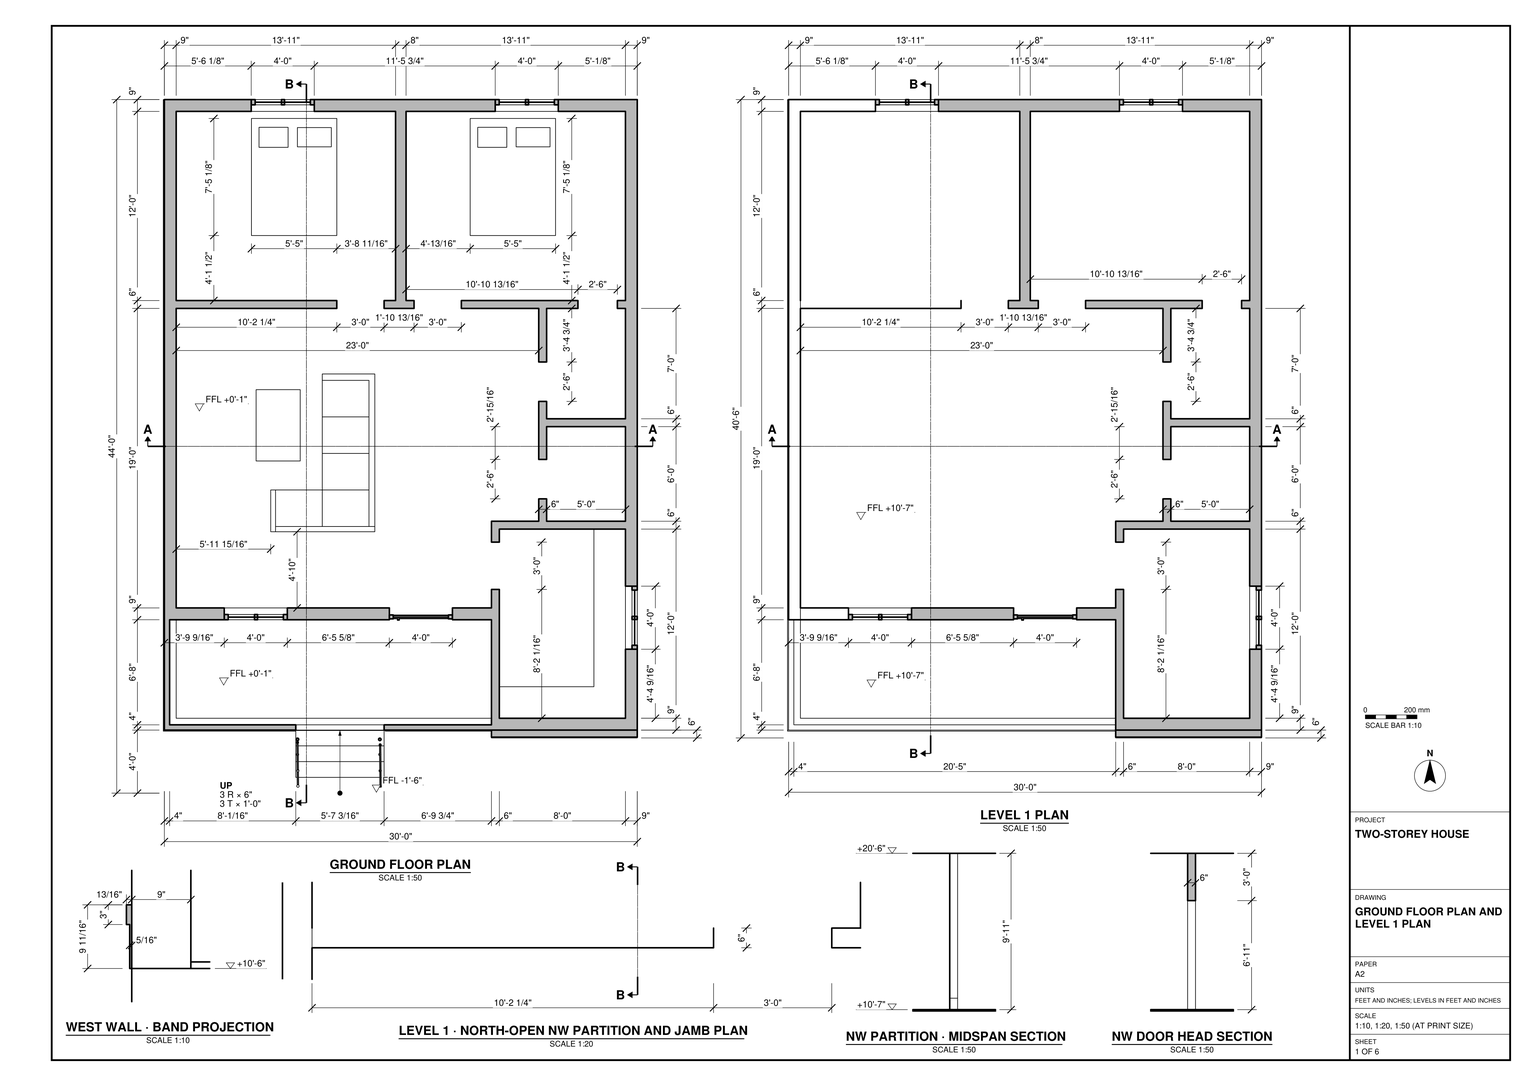
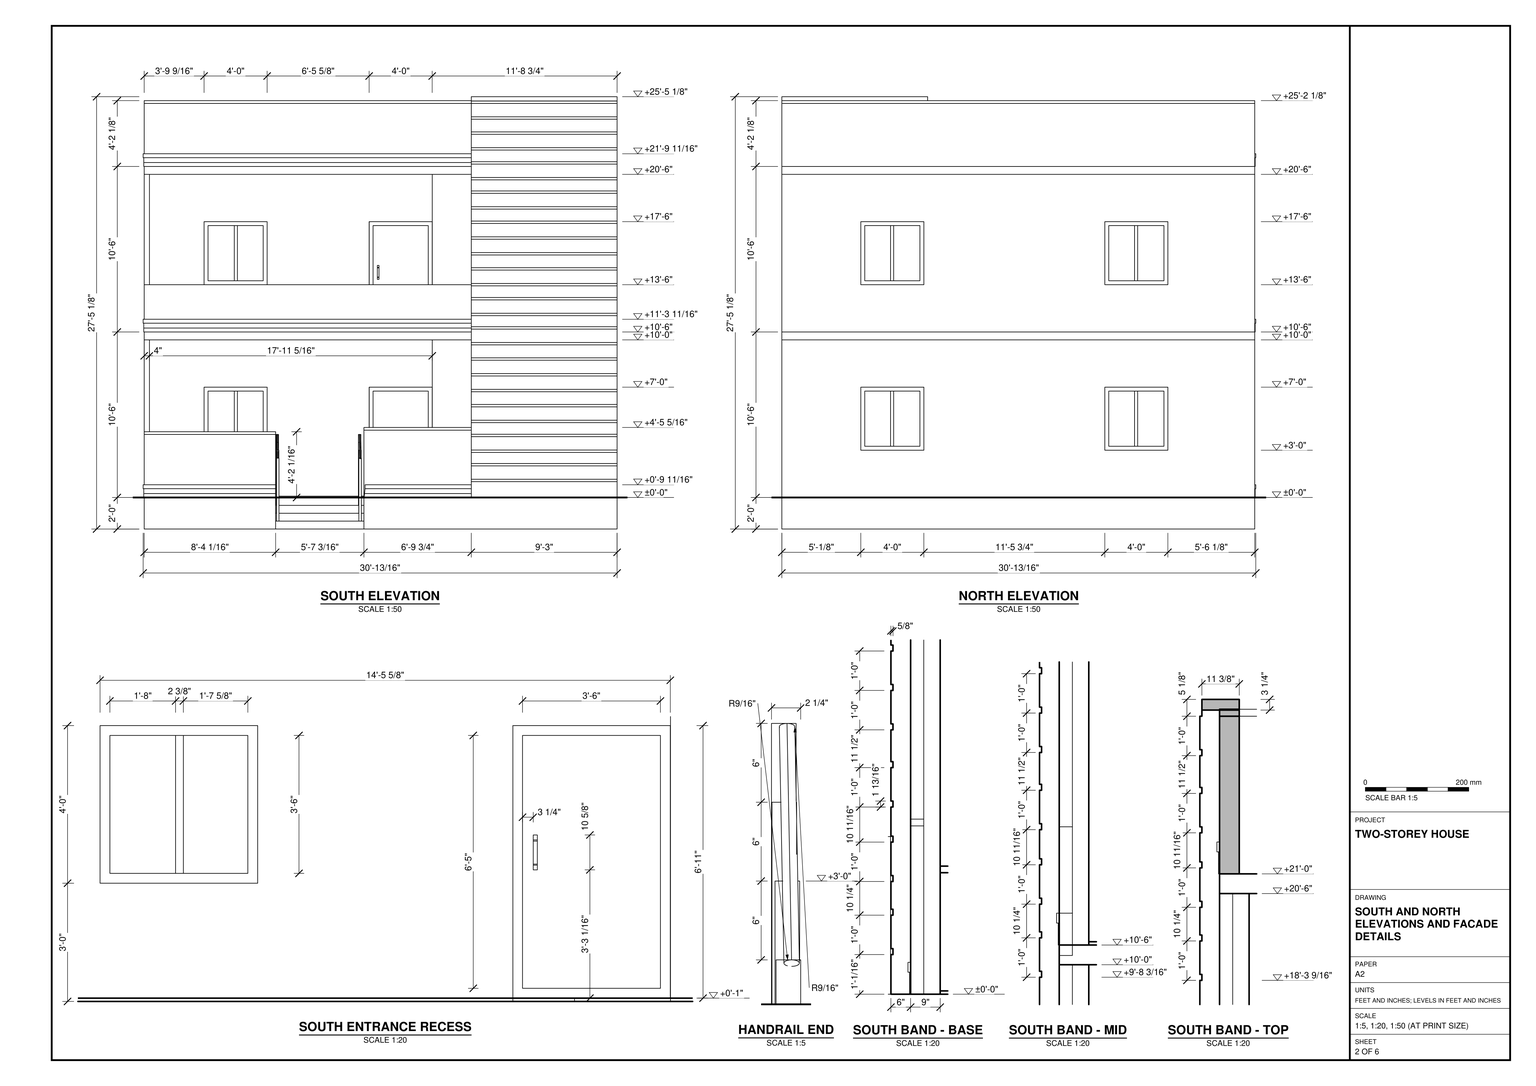
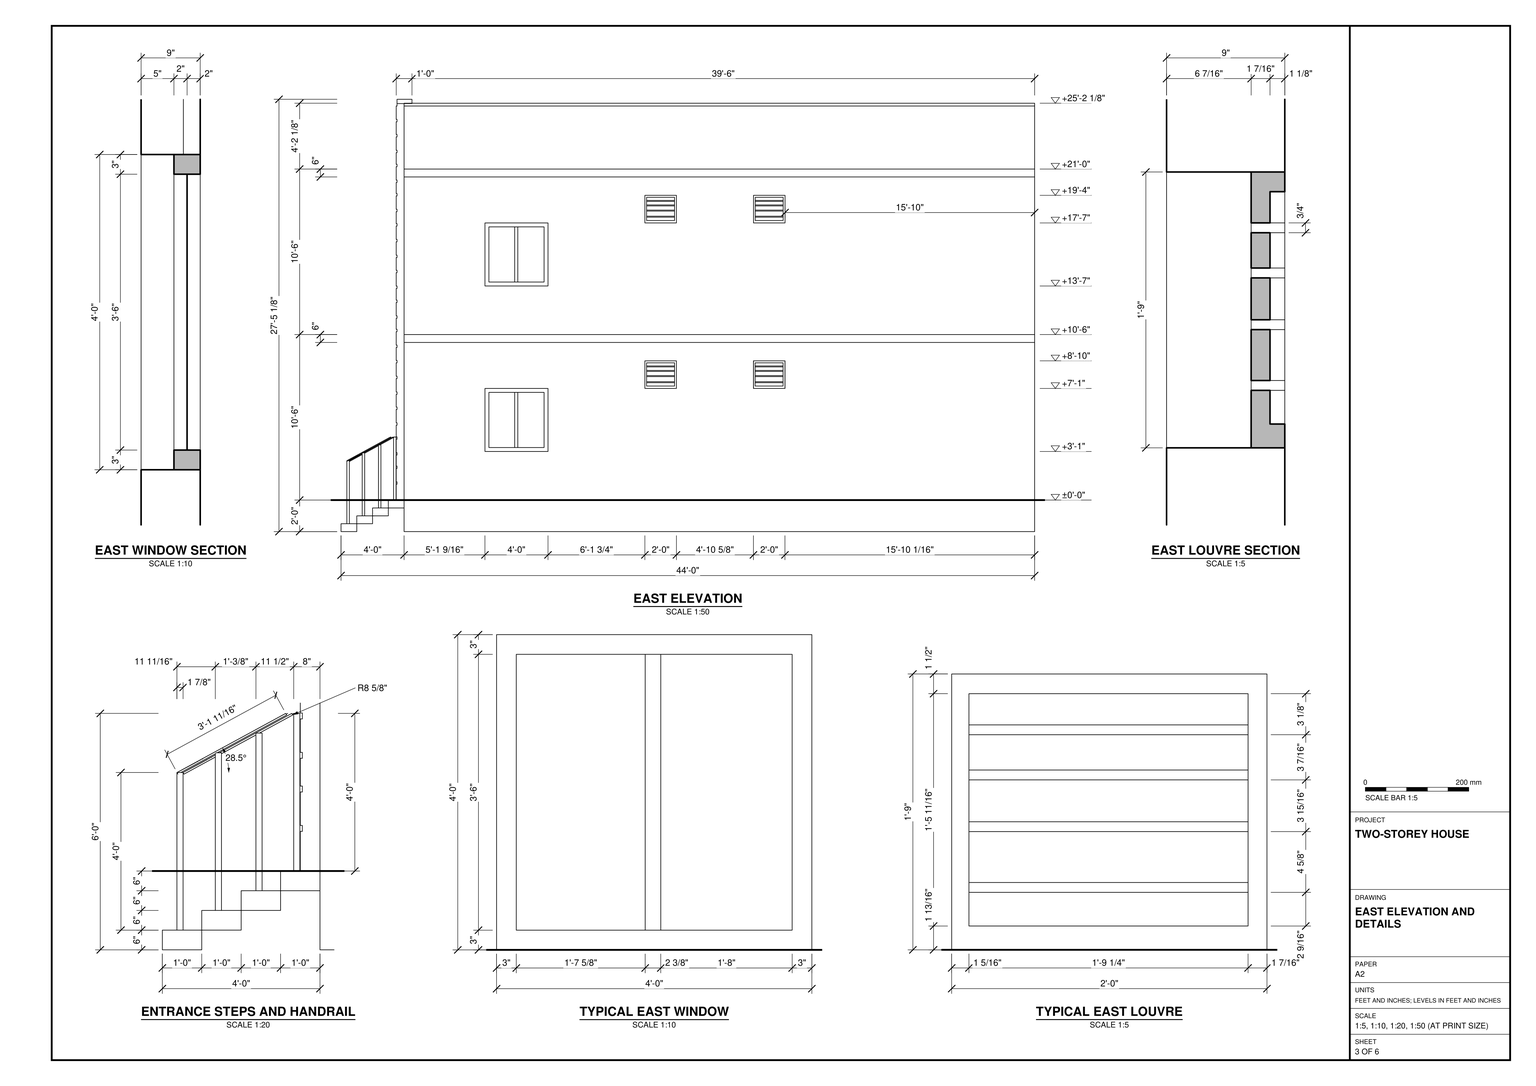
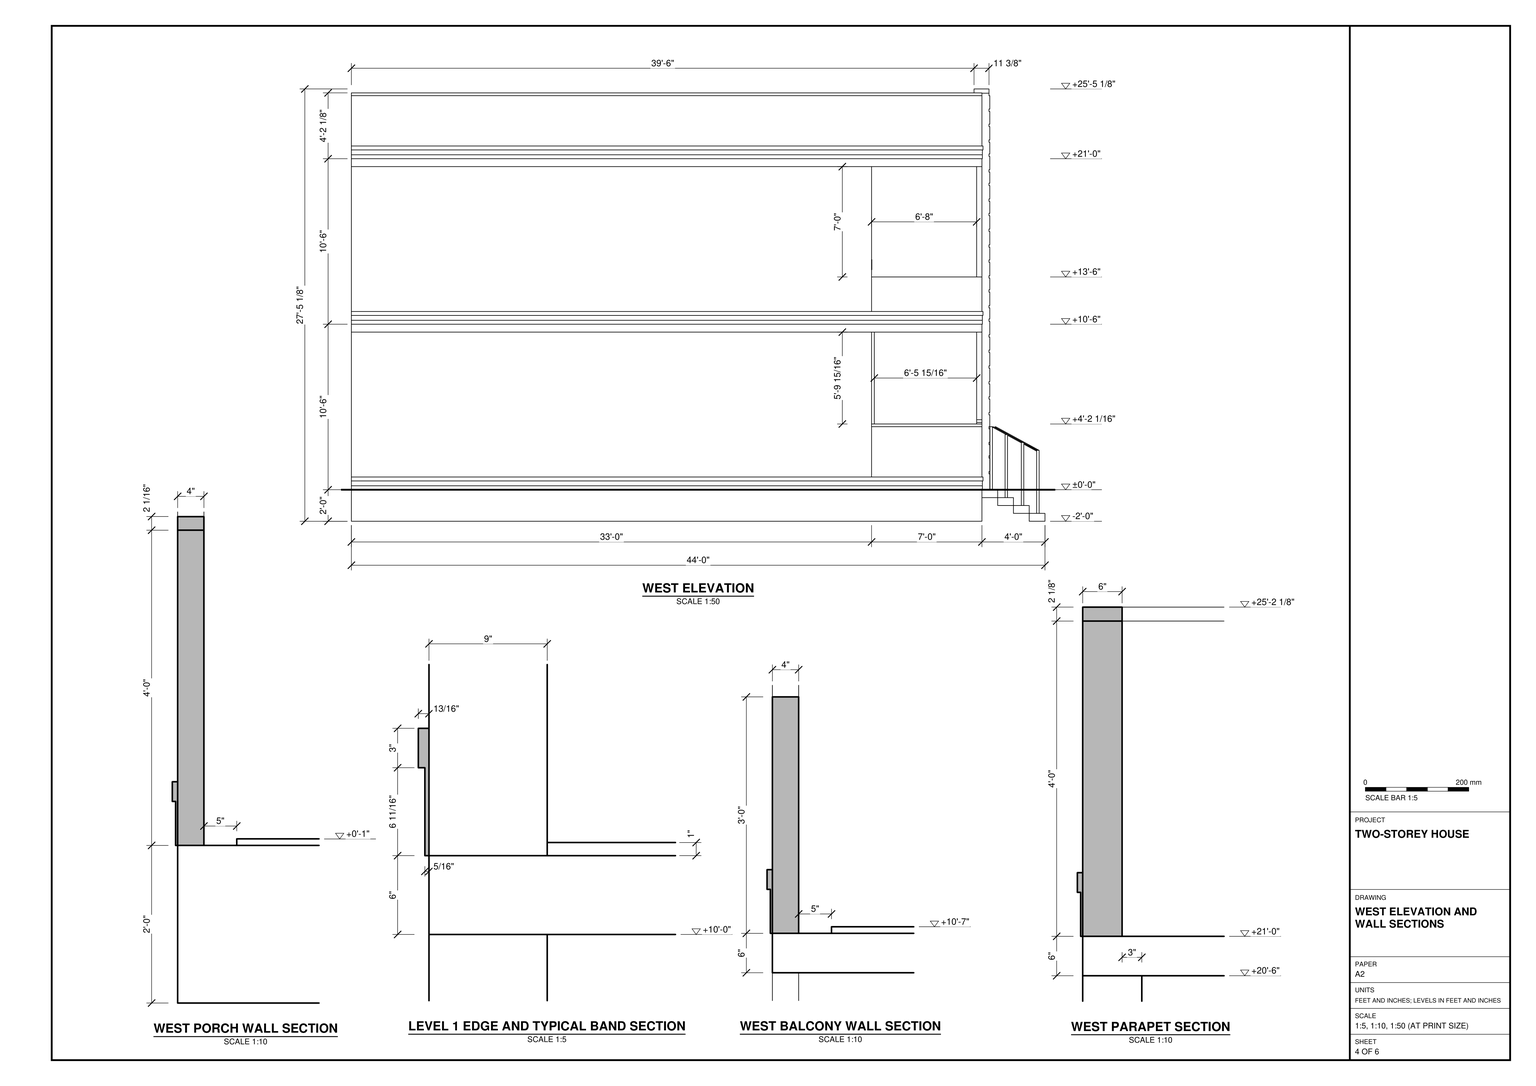
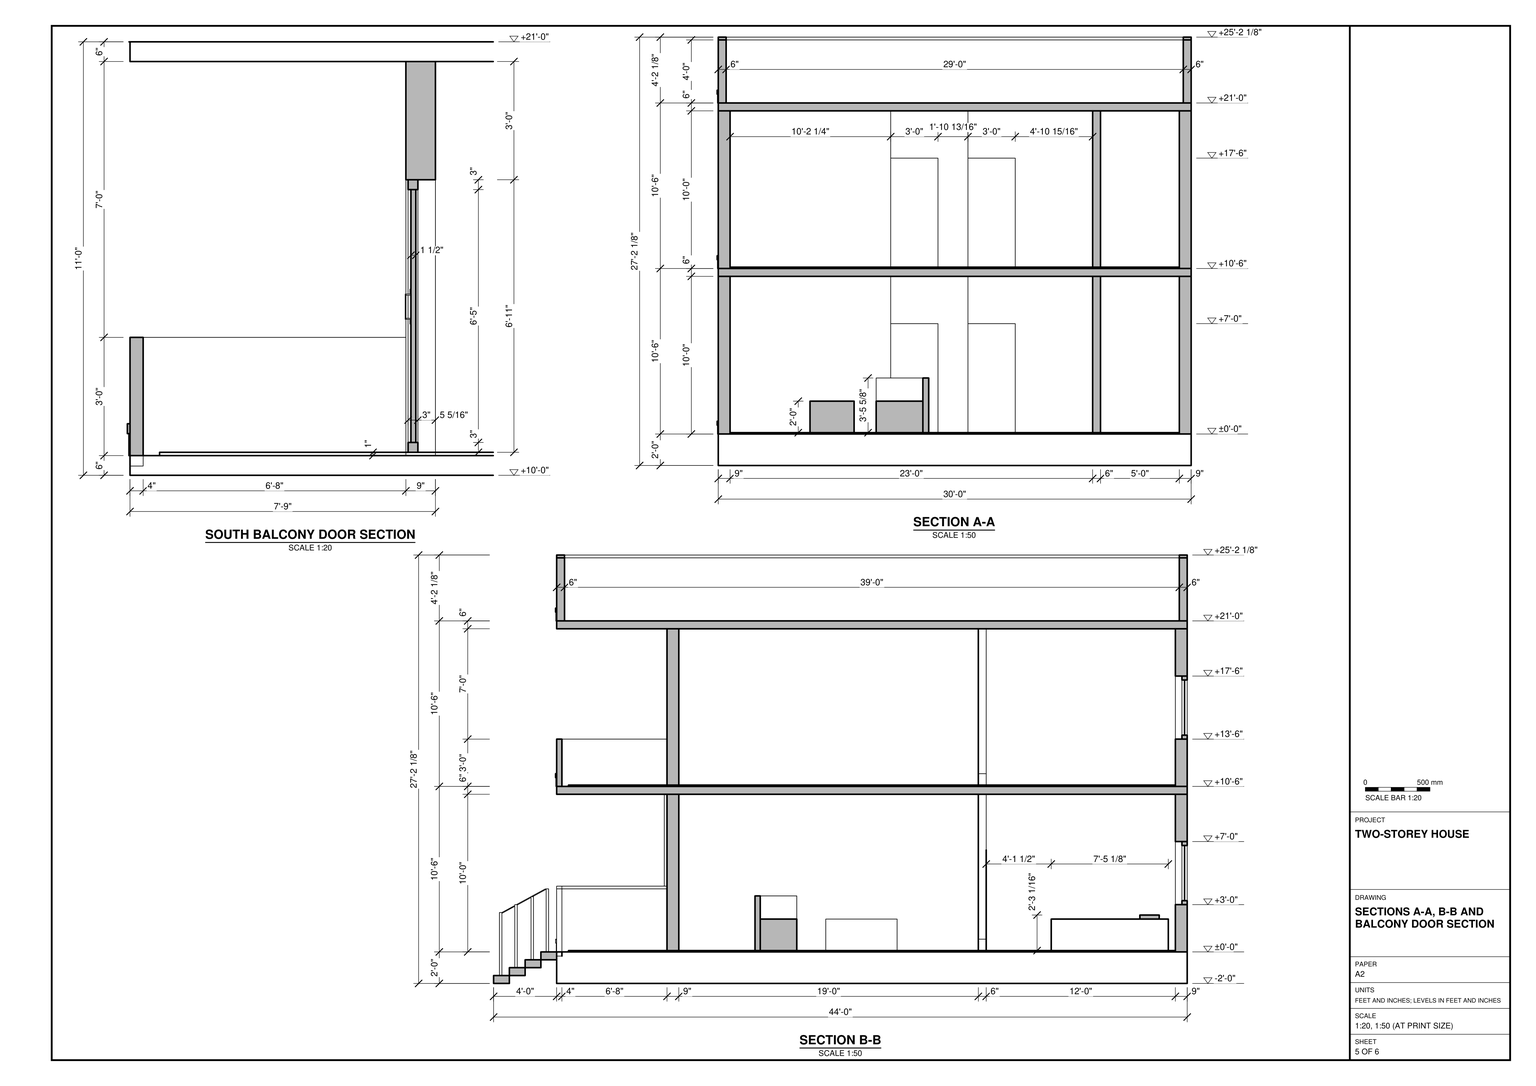
Build the house in SketchUp using task_files/diagram_01.pdf. Work in feet and inches. The overall model measures 30'-13/16" east to west, 44'-0" north to south including the entrance steps, and 27'-5 1/8" from its lowest point to its highest point. Set the ground floor at ±0'-0" and the upper floor at +10'-6".

Use the two plans separately to lay out the walls and openings. Follow the drawn wall thicknesses, including the 9" exterior walls, the 8" dividing wall between the rear rooms and the 6" partitions where indicated. Follow the upper-floor partition and jamb detail at the northwest room. Model the floor slabs, flat roof and parapets. On the south side, form the recessed porch and the balcony above it, with the entrance steps and handrails leading through the gap in the porch wall. Carry the horizontal bands across the full-height bay beside the recess as shown in elevation.

Fit the doors, window units and east-wall louvres to their openings. Place the beds in the rear ground-floor rooms and arrange the L-shaped sofa and low table to match their plan footprints. Decor and loose items may be any suitable library components. Keep walls, slabs, roof, and each furniture or joinery piece in separate groups or components, and use components for repeated parts. Save one SketchUp model as output_files/two_storey_house_with_a_recessed_porch_and_balcony.skp.

# SketchUp Ruby script. Lengths in inches.
U = 1.inch
M = Sketchup.active_model
def pt(a) = Geom::Point3d.new(a.map { |v| v * U })
def face(e, loops, mat)
  f = e.add_face(loops[0].map { |a| pt(a) })
  loops[1..].each { |l| e.add_face(l.map { |a| pt(a) }).erase! }
  f.material = f.back_material = mat if mat
  f
end
# faces: each face lists its corners as indices into pts; further lists are holes
def faces(e, pts, list, mat = nil) = list.each { |f| face(e, (f[0].is_a?(Array) ? f : [f]).map { |l| l.map { |i| pts[i] } }, mat) }
# xy, xz, yz: faces in a plane at the given z, y or x. An outline is a flat list of corners, or four numbers for a rectangle; further outlines are holes
def ring(l) = l.size == 4 ? [[l[0], l[1]], [l[2], l[1]], [l[2], l[3]], [l[0], l[3]]] : l.each_slice(2).to_a
def flat(e, list, mat, &to3) = list.each { |f| face(e, (f[0].is_a?(Array) ? f : [f]).map { |l| ring(l).map { |u, v| to3.(u, v) } }, mat) }
def xy(e, z, list, mat = nil) = flat(e, list, mat) { |x, y| [x, y, z] }
def xz(e, y, list, mat = nil) = flat(e, list, mat) { |x, z| [x, y, z] }
def yz(e, x, list, mat = nil) = flat(e, list, mat) { |y, z| [x, y, z] }
def lines(e, pts, list) = list.each { |a, b| e.add_line(pt(pts[a]), pt(pts[b])) }
# prism: a flat outline (further loops are holes) pulled along v
def prism(e, loops, v, mat = nil)
  f = face(e, loops, mat); d = Geom::Vector3d.new(v.map { |x| x * U })
  f.pushpull(f.normal.samedirection?(d) ? d.length : -d.length)
end
def box(e, o, s, mat = nil) = prism(e, [[o, [o[0] + s[0], o[1], o[2]], [o[0] + s[0], o[1] + s[1], o[2]], [o[0], o[1] + s[1], o[2]]]], [0, 0, s[2]], mat)
def at(x, y, z, deg = 0) = Geom::Transformation.translation(pt([x, y, z])) * Geom::Transformation.rotation(ORIGIN, Z_AXIS, deg.degrees)
def axes(o, x, y, z) = Geom::Transformation.new([*x, 0, *y, 0, *z, 0, *pt(o).to_a, 1])
def part(name) = M.definitions.add(name)
# library, detail: a bought-in or finely detailed component or shape, given as its bounding box
def library(name, o, s) = part(name).tap { |d| box(d.entities, o, s) }
def detail(e, o, s) = box(e.add_group.entities, o, s)
def put(e, d, t, mat = nil) = e.add_instance(d, t).tap { |i| i.material = mat if mat }
def group(e, t, mat = nil) = e.add_group.tap { |g| g.transformation = t; g.material = mat if mat }.entities
root = M.entities
M.materials.add("A01_Blush_Petal").color = [255, 204, 204]
M.materials.add("A02_Rose_Quartz").color = [255, 153, 153]
M.materials.add("C07_Caramel_Shine").color = [153, 76, 0]
M.materials.add("C08_Toffee_Ember").color = [102, 51, 0]
M.materials.add("D01_Frost_White").color = [255, 242, 206]
M.materials.add("D02_Buttercup_Glow").color = [255, 229, 155]
M.materials.add("D03_Lemon_Mist").color = [255, 216, 101]
M.materials.add("Forest_Floor_01_1K").color = [106, 91, 72]
M.materials.add("Glass_Basic_01").color = [161, 173, 186]
M.materials["Glass_Basic_01"].alpha = 0.25
M.materials.add("Glass_Safety_01").color = [204, 235, 244]
M.materials["Glass_Safety_01"].alpha = 0.25
M.materials.add("H02_Aqua_Frost").color = [153, 255, 255]
M.materials.add("H07_Deep_Teal").color = [0, 153, 153]
M.materials.add("M01_Silver_Fog").color = [224, 224, 224]
M.materials.add("M05_Graphite_Haze").color = [114, 114, 114]
M.materials.add("M09_Shadow_Night").color = [0, 0, 0]
M.materials.add("Marble_06_1K").color = [165, 150, 147]
M.materials.add("Metal_06_1K").color = [238, 236, 231]
M.materials.add("Plywood_01_1K").color = [125, 96, 64]
c1 = part("Group\#5")
box(c1.entities,[-7.22,0,-6],[67.22,12,6])
c2 = part("Group\#9")
g1 = group(c2.entities,at(3,2,3),"Glass_Safety_01")
xz(g1,0,[[0,0,42,42]])
g2 = group(c2.entities,at(0,4,0),"Plywood_01_1K")
xy(g2,0,[[0,-4,48,0]])
xy(g2,3,[[3,-4,23,0],[23,-4,25.375,0],[25.375,-4,45,0]])
xy(g2,45,[[3,-4,23,0],[23,-4,25.375,0],[25.375,-4,45,0]])
xy(g2,48,[[0,-4,48,0]])
xz(g2,-4,[[[0,0,48,48],[3,3,45,45]],[23,3,25.375,45]],"Plywood_01_1K")
xz(g2,0,[[[0,0,48,48],[3,3,45,45]],[23,3,25.375,45]])
yz(g2,0,[[-4,0,0,48]])
yz(g2,3,[[-4,3,0,45]])
yz(g2,23,[[-4,3,0,45]])
yz(g2,25.375,[[-4,3,0,45]])
yz(g2,45,[[-4,3,0,45]])
yz(g2,48,[[-4,0,0,48]])
c3 = part("Group\#10")
xy(c3.entities,0,[[-0.25,0,2.3125,24]])
xy(c3.entities,1.8125,[[1.1875,1.3125,2.3125,22.5625]])
xy(c3.entities,4.375,[[-0.25,1.3125,1.1875,22.5625]])
xy(c3.entities,5.125,[[-0.25,1.3125,1.1875,22.5625]])
xy(c3.entities,9,[[-0.25,1.3125,1.1875,22.5625]])
xy(c3.entities,9.75,[[-0.25,1.3125,1.1875,22.5625]])
xy(c3.entities,12.9375,[[-0.25,1.3125,1.1875,22.5625]])
xy(c3.entities,13.6875,[[-0.25,1.3125,1.1875,22.5625]])
xy(c3.entities,16.375,[[-0.25,1.3125,1.1875,22.5625]])
xy(c3.entities,17.125,[[-0.25,1.3125,1.1875,22.5625]])
xy(c3.entities,19.5,[[1.1875,1.3125,2.3125,22.5625]])
xy(c3.entities,21,[[-0.25,0,2.3125,24]])
xz(c3.entities,0,[[-0.25,0,2.3125,21]])
xz(c3.entities,1.3125,[[1.1875,1.8125,2.3125,4.375],[-0.25,4.375,2.3125,5.125],[1.1875,5.125,2.3125,9],[-0.25,9,2.3125,9.75],[1.1875,9.75,2.3125,12.9375],
  [-0.25,12.9375,2.3125,13.6875],[1.1875,13.6875,2.3125,16.375],[-0.25,16.375,2.3125,17.125],[1.1875,17.125,2.3125,19.5]])
xz(c3.entities,22.5625,[[1.1875,1.8125,2.3125,4.375],[-0.25,4.375,2.3125,5.125],[1.1875,5.125,2.3125,9],[-0.25,9,2.3125,9.75],[1.1875,9.75,2.3125,12.9375],
  [-0.25,12.9375,2.3125,13.6875],[1.1875,13.6875,2.3125,16.375],[-0.25,16.375,2.3125,17.125],[1.1875,17.125,2.3125,19.5]])
xz(c3.entities,24,[[-0.25,0,2.3125,21]])
yz(c3.entities,-0.25,[[[0,0,24,21],[1.3125,16.375,22.5625,17.125],[1.3125,12.9375,22.5625,13.6875],[1.3125,9,22.5625,9.75],[1.3125,4.375,22.5625,5.125]]])
yz(c3.entities,1.1875,[[1.3125,1.8125,22.5625,4.375],[1.3125,5.125,22.5625,9],[1.3125,9.75,22.5625,12.9375],[1.3125,13.6875,22.5625,16.375],[1.3125,17.125,22.5625,19.5]])
yz(c3.entities,2.3125,[[[0,0,24,21],[1.3125,1.8125,22.5625,19.5]]])
c4 = part("Group\#16")
g3 = group(c4.entities,at(0,3.875,0),"Plywood_01_1K")
prism(g3,[[[0,0,83],[48,0,83],[48,0,0],[0,0,0]],[[45,0,3],[45,0,80],[3,0,80],[3,0,3]]],[0,-3,0])
g4 = group(c4.entities,at(6.26,1.75,47.9375),"Metal_06_1K")
xy(g4,-8.875,[[0,-0.3125,1.25,0]])
xy(g4,-7.4375,[[0,-1.75,1.25,-1.5],[0,-1.5,1.25,-0.3125],[0,-0.3125,1.25,0]])
xy(g4,-7.125,[[0,-1.75,1.25,-1.5],[0,-1.5,1.25,0]])
xy(g4,-0.125,[[0,-1.75,1.25,-1.5],[0,-1.5,1.25,0]])
xy(g4,0.25,[[0,-1.75,1.25,-1.5],[0,-1.5,1.25,-0.3125],[0,-0.3125,1.25,0]])
xy(g4,1.75,[[0,-0.3125,1.25,0]])
xz(g4,-1.75,[[0,-7.4375,1.25,-7.125],[0,-7.125,1.25,-0.125],[0,-0.125,1.25,0.25]])
xz(g4,-1.5,[[0,-7.4375,1.25,-7.125],[0,-7.125,1.25,-0.125],[0,-0.125,1.25,0.25]])
xz(g4,-0.3125,[[0,-8.875,1.25,-7.4375],[0,0.25,1.25,1.75]])
xz(g4,0,[[0,-7.4375,1.25,-7.125],[0,-0.125,1.25,0.25],[0,0.25,1.25,1.75]])
yz(g4,0,[[-0.3125,-8.875,0,-7.4375],[-1.75,-7.4375,-1.5,-7.125],[-1.5,-7.4375,0,-7.125],[-1.75,-7.125,-1.5,-0.125],[-1.75,-0.125,-1.5,0.25],
  [-1.5,-0.125,0,0.25],[-0.3125,0.25,0,1.75]])
yz(g4,1.25,[[-0.3125,-8.875,0,-7.4375],[-1.75,-7.4375,-1.5,-7.125],[-1.5,-7.4375,0,-7.125],[-1.75,-7.125,-1.5,-0.125],[-1.75,-0.125,-1.5,0.25],
  [-1.5,-0.125,0,0.25],[-0.3125,0.25,0,1.75]])
g5 = group(c4.entities,at(3,3.25,3))
box(g5,[0,-1.5,0],[42,1.5,77],"Plywood_01_1K")
c5 = part("Group\#19")
prism(c5.entities,[[[0.9375,1.875,0],[1.18,1.84,0],[1.41,1.75,0],[1.6,1.6,0],[1.75,1.41,0],[1.84,1.18,0],[1.875,0.9375,0],[1.84,0.69,0],[1.75,0.47,0],[1.6,0.27,0],[1.41,0.125,0],[1.18,0.03,0],[0.9375,0,0],[0.69,0.03,0],[0.47,0.125,0],[0.27,0.27,0],[0.125,0.47,0],[0.03,0.69,0],[0,0.9375,0],[0.03,1.18,0],[0.125,1.41,0],[0.27,1.6,0],[0.47,1.75,0],[0.69,1.84,0]]],[0,0,48])
c6 = part("Group\#20")
prism(c6.entities,[[[1.24,-32.84,-18.46],[1.36,-32.86,-18.42],[1.46,-32.89,-18.37],[1.51,-32.92,-18.31],[1.53,-32.95,-18.24],[1.51,-32.99,-18.18],[1.45,-33.02,-18.12],[1.36,-33.05,-18.07],[1.23,-33.07,-18.03],[1.09,-33.09,-18.01],[0.9375,-33.09,-18],[0.79,-33.09,-18.01],[0.64,-33.08,-18.03],[0.52,-33.06,-18.07],[0.43,-33.03,-18.125],[0.37,-33,-18.1875],[0.35,-32.96,-18.25],[0.375,-32.93,-18.3125],[0.44,-32.9,-18.375],[0.53,-32.87,-18.42],[0.65,-32.84,-18.46],[0.8,-32.83,-18.49],[0.95,-32.82,-18.49],[1.1,-32.83,-18.49]]],[-0.35,33.09,18])
c7 = part("Group\#22")
xy(c7.entities,0,[[-0.3125,-0.3125,0,480],[0,-0.3125,249,0]],"C08_Toffee_Ember")
xy(c7.entities,6.69,[[-0.8125,-0.8125,-0.3125,480],[-0.3125,-0.8125,249,-0.3125]],"C08_Toffee_Ember")
xy(c7.entities,9.69,[[-0.8125,-0.8125,249,0],[-0.8125,0,0,480]],"C08_Toffee_Ember")
xz(c7.entities,-0.8125,[[-0.8125,6.69,249,9.69]],"C08_Toffee_Ember")
xz(c7.entities,-0.3125,[[-0.3125,0,249,3]],"C08_Toffee_Ember")
xz(c7.entities,-0.3125,[[-0.3125,3,249,6.69]],"D03_Lemon_Mist")
xz(c7.entities,480,[[-0.3125,3,0,6.69]])
xz(c7.entities,480,[[-0.3125,0,0,3],[-0.8125,6.69,0,9.69]],"C08_Toffee_Ember")
yz(c7.entities,-0.8125,[[-0.8125,6.69,480,9.69]],"C08_Toffee_Ember")
yz(c7.entities,-0.3125,[[-0.3125,0,480,3]],"C08_Toffee_Ember")
yz(c7.entities,-0.3125,[[-0.3125,3,480,6.69]],"D03_Lemon_Mist")
yz(c7.entities,249,[[-0.3125,3,0,6.69]])
yz(c7.entities,249,[[-0.3125,0,0,3],[-0.8125,6.69,0,9.69]],"C08_Toffee_Ember")
c8 = part("Group\#28")
box(c8.entities,[0,0,0],[35.5625,27.8125,24])
c9 = part("Group\#30")
box(c9.entities,[0,0,0],[65,89.125,24])
g6 = group(c9.entities,at(5.77,67.15,24),"A02_Rose_Quartz")
box(g6,[29.21,0.36,0],[25.82,14.69,3.0625])
box(g6,[0,0,0],[22.125,15.25,3.0625])
xy(root,1,[[70.66,252.86,104.22,307.17]])
xy(root,25,[[70.66,252.86,104.22,307.17]],"A01_Blush_Petal")
xy(root,252,[[6.8125,54,354.8125,522]])
xz(root,252.86,[[70.66,1,104.22,25]],"Glass_Basic_01")
xz(root,307.17,[[70.66,1,104.22,25]],"Glass_Basic_01")
xz(root,375,[[9.8125,0,132.08,77.62]])
yz(root,70.66,[[252.86,1,307.17,25]],"Glass_Basic_01")
yz(root,104.22,[[252.86,1,307.17,25]],"Glass_Basic_01")
p = [[100.87,48,0],[108.08,48,0]]
lines(root,p,[[0,1]])
g7 = group(root,at(0.8125,48,0))
xy(g7,0,[[0,0,100.05,0,100.05,4,4,4,4,84,0,84],[249,0,360,0,360,480,0,480,0,84,45.59,84,45.59,93,9,93,9,321,131.27,321,131.27,327,9,327,9,471,176,471,176,327,167.27,327,167.27,321,190.08,321,190.08,327,184,327,184,471,351,471,351,327,344.84,327,344.84,321,351,321,351,237,291,237,291,321,314.84,321,314.84,327,226.08,327,226.08,321,285,321,285,206.03,291,206.03,291,231,351,231,351,159,291,159,291,176.03,285,176.03,285,159,249,159,249,143.07,255,143.07,255,153,351,153,351,9,255,9,255,107.07,249,107.07,249,93,219.3,93,219.3,84,249,84],[167.27,0,249,4],[255,9,351,153],[45.59,84,93.59,93],
  [93.59,84,171.3,93],[171.3,84,219.3,93],[9,93,249,93,249,159,285,159,285,321,9,321],[249,107.07,255,143.07],[291,159,351,231],
  [285,176.03,291,206.03],[291,237,351,321],[131.27,321,167.27,327],[190.08,321,226.08,327],[314.84,321,344.84,327],
  [9,327,176,471],[184,327,351,471]])
xy(g7,0,[[100.05,0,167.27,4],[4,4,249,84]],"D02_Buttercup_Glow")
g8 = group(root,at(0.8125,48,120),"D01_Frost_White")
box(g8,[0,0,0],[360,480,6])
g9 = group(root,at(0.8125,48,0),"D01_Frost_White")
xy(g9,0,[[0,0,0,84,4,84,4,4,100.05,4,100.05,0],[45.59,84,171.3,93],[285,250.22,291,280.22]])
xy(g9,36,[[45.59,84,93.59,93],[66.125,471,114.125,480],[251.875,471,299.875,480]])
xy(g9,37,[[351,61.5625,360,109.5625]])
xy(g9,48,[[0,0,0,84,4,84,4,4,100.05,4,100.05,0]],"M05_Graphite_Haze")
xy(g9,50.0625,[[0,0,100.05,0,100.05,4,4,4,4,81.9375,0,81.9375],[0,81.9375,4,84]],"M05_Graphite_Haze")
xy(g9,51.25,[[167.27,0,249,4]],"M05_Graphite_Haze")
xy(g9,53.3125,[[167.27,0,249,4]],"M05_Graphite_Haze")
xy(g9,84,[[45.59,84,93.59,93],[171.3,84,219.3,93],[249,107.07,255,143.07],[285,176.03,291,206.03],[285,250.22,291,280.22],
  [131.27,321,167.27,327],[190.08,321,226.08,327],[314.84,321,344.84,327],[66.125,471,114.125,480],[251.875,471,299.875,480]])
xy(g9,85,[[351,61.5625,360,109.5625],[351,183.3125,360,207.3125],[351,266,360,290]])
xy(g9,106,[[351,183.3125,360,207.3125],[351,266,360,290]])
xy(g9,120,[[[249,0,360,0,360,480,0,480,0,84,219.3,84,219.3,93,9,93,9,321,131.27,321,131.27,327,9,327,9,471,176,471,176,327,131.27,327,131.27,321,285,321,285,206.03,291,206.03,291,231,351,231,351,159,291,159,291,206.03,285,206.03,285,159,249,159,249,143.07,255,143.07,255,153,351,153,351,9,255,9,255,143.07,249,143.07,249,93,219.3,93,219.3,84,249,84],[291,237,291,321,314.84,321,314.84,327,184,327,184,471,351,471,351,327,314.84,327,314.84,321,351,321,351,237]]])
xy(g9,120,[[0,81.9375,4,84]],"M05_Graphite_Haze")
xz(g9,0,[[0,0,100.05,48],[167.27,0,249,51.25],[249,0,360,120]])
xz(g9,0,[[0,48,100.05,50.0625],[167.27,51.25,249,53.3125]],"M05_Graphite_Haze")
xz(g9,4,[[100.05,-3.1875,167.27,0],[4,0,100.05,48],[167.27,0,249,51.25]])
xz(g9,4,[[4,48,100.05,50.0625],[167.27,51.25,249,53.3125]],"M05_Graphite_Haze")
xz(g9,9,[[255,0,351,120]])
xz(g9,61.5625,[[351,37,360,85]])
xz(g9,81.9375,[[0,50.0625,4,120]],"M05_Graphite_Haze")
xz(g9,84,[[[4,0,171.3,0,171.3,84,219.3,84,219.3,120,4,120],[45.59,36,93.59,84]],[219.3,0,249,120]])
xz(g9,84,[[0,48,4,50.0625],[0,50.0625,4,120]],"M05_Graphite_Haze")
xz(g9,93,[[[9,0,9,120,219.3,120,219.3,84,171.3,84,171.3,0],[45.59,36,93.59,84]],[219.3,0,249,120]])
xz(g9,107.07,[[249,0,255,84]])
xz(g9,109.5625,[[351,37,360,85]])
xz(g9,143.07,[[249,0,255,84]])
xz(g9,153,[[255,0,351,120]])
xz(g9,159,[[249,0,285,120],[291,0,351,120]])
xz(g9,176.03,[[285,0,291,84]])
xz(g9,183.3125,[[351,85,360,106]])
xz(g9,206.03,[[285,0,291,84]])
xz(g9,207.3125,[[351,85,360,106]])
xz(g9,231,[[291,0,351,120]])
xz(g9,237,[[291,0,351,120]])
xz(g9,250.22,[[285,0,291,84]])
xz(g9,266,[[351,85,360,106]])
xz(g9,280.22,[[285,0,291,84]])
xz(g9,290,[[351,85,360,106]])
xz(g9,321,[[9,0,131.27,120],[167.27,0,190.08,0,190.08,120,131.27,120,131.27,84,167.27,84],[226.08,0,285,0,285,120,190.08,120,190.08,84,226.08,84],[291,0,314.84,120],[344.84,0,351,0,351,120,314.84,120,314.84,84,344.84,84]])
xz(g9,327,[[167.27,0,167.27,84,131.27,84,131.27,120,176,120,176,0],[184,0,190.08,120],[226.08,0,226.08,84,190.08,84,190.08,120,314.84,120,314.84,0],[344.84,0,344.84,84,314.84,84,314.84,120,351,120,351,0]])
xz(g9,471,[[[9,0,176,120],[66.125,36,114.125,84]],[[184,0,351,120],[251.875,36,299.875,84]]])
xz(g9,480,[[[0,0,360,120],[66.125,36,114.125,84],[251.875,36,299.875,84]]])
yz(g9,0,[[0,0,84,48],[84,0,480,120]])
yz(g9,0,[[0,48,84,50.0625],[81.9375,50.0625,84,120]],"M05_Graphite_Haze")
yz(g9,4,[[4,0,84,48]])
yz(g9,4,[[4,48,84,50.0625],[81.9375,50.0625,84,120]],"M05_Graphite_Haze")
yz(g9,9,[[93,0,321,120],[327,0,471,120]])
yz(g9,45.59,[[84,36,93,84]])
yz(g9,66.125,[[471,36,480,84]])
yz(g9,93.59,[[84,36,93,84]])
yz(g9,100.05,[[0,-3.1875,4,0],[0,0,4,48]])
yz(g9,100.05,[[0,48,4,50.0625]],"M05_Graphite_Haze")
yz(g9,114.125,[[471,36,480,84]])
yz(g9,131.27,[[321,0,327,84]])
yz(g9,167.27,[[0,-3.1875,4,51.25],[321,0,327,84]])
yz(g9,167.27,[[0,51.25,4,53.3125]],"M05_Graphite_Haze")
yz(g9,171.3,[[84,0,93,84]])
yz(g9,176,[[327,0,471,120]])
yz(g9,184,[[327,0,471,120]])
yz(g9,190.08,[[321,0,327,84]])
yz(g9,219.3,[[84,0,93,84]])
yz(g9,226.08,[[321,0,327,84]])
yz(g9,249,[[4,0,84,120],[93,0,93,120,143.07,120,143.07,84,107.07,84,107.07,0],[143.07,0,159,120],[0,53.3125,4,120]])
yz(g9,249,[[0,51.25,4,53.3125]],"M05_Graphite_Haze")
yz(g9,251.875,[[471,36,480,84]])
yz(g9,255,[[9,0,107.07,0,107.07,84,143.07,84,143.07,120,9,120],[143.07,0,153,120]])
yz(g9,285,[[159,0,159,120,206.03,120,206.03,84,176.03,84,176.03,0],[206.03,0,250.22,120],[280.22,0,280.22,84,250.22,84,250.22,120,321,120,321,0]])
yz(g9,291,[[159,0,176.03,0,176.03,84,206.03,84,206.03,120,159,120],[206.03,0,231,120],[237,0,250.22,120],[280.22,0,321,0,321,120,250.22,120,250.22,84,280.22,84]])
yz(g9,299.875,[[471,36,480,84]])
yz(g9,314.84,[[321,0,327,84]])
yz(g9,344.84,[[321,0,327,84]])
yz(g9,351,[[[9,0,153,120],[61.5625,37,109.5625,85]],[[159,0,231,120],[183.3125,85,207.3125,106]],[[237,0,321,120],[266,85,290,106]],[327,0,471,120]])
yz(g9,360,[[[0,0,480,120],[61.5625,37,109.5625,85],[183.3125,85,207.3125,106],[266,85,290,106]]])
g10 = group(root,at(0.8125,-129.8125,-24),"D02_Buttercup_Glow")
xy(g10,0,[[0,177.8125,360,657.8125]])
xy(g10,24,[[0,177.8125,360,657.8125]])
xz(g10,177.8125,[[0,0,360,24]],"M05_Graphite_Haze")
xz(g10,657.8125,[[0,0,360,24]],"M05_Graphite_Haze")
yz(g10,0,[[177.8125,0,657.8125,24]],"M05_Graphite_Haze")
yz(g10,360,[[177.8125,0,657.8125,24]],"M05_Graphite_Haze")
put(root,c1,at(108.08,36,0),"Forest_Floor_01_1K")
put(root,c1,at(108.08,24,-6),"Forest_Floor_01_1K")
put(root,c1,at(108.08,12,-12),"Forest_Floor_01_1K")
put(root,c1,at(108.08,0,-18),"Forest_Floor_01_1K")
g11 = group(root,at(9.8125,57,0),"Marble_06_1K")
prism(g11,[[[0,318,0],[0,462,0],[342,462,0],[342,0,0],[0,0,0]]],[0,0,1])
p = [[246.01,24,1],[318,24,1],[318,143.6875,1]]
lines(g11,p,[[0,1],[1,2]])
put(root,c2,at(46.4,132,36))
put(root,c2,at(252.6875,524,36))
put(root,c2,at(66.9375,524,36))
put(root,c2,at(356.8125,157.5625,37,-90))
put(root,c3,at(358.5,231.3125,85),"D02_Buttercup_Glow")
put(root,c3,at(358.5,313.9375,85),"D02_Buttercup_Glow")
g12 = group(root,at(0.8125,48,126),"D01_Frost_White")
xy(g12,0,[[0,0,0,84,4,84,4,4,100.05,4,100.05,0],[45.59,84,171.3,93],[285,250.22,291,280.22]])
xy(g12,36,[[45.59,84,93.59,93],[66.125,471,114.125,480],[251.875,471,299.875,480]])
xy(g12,36,[[0,0,249,0,249,4,4,4,4,84,0,84]],"M05_Graphite_Haze")
xy(g12,37,[[351,61.5625,360,109.5625]])
xy(g12,84,[[45.59,84,93.59,93],[171.3,84,219.3,93],[249,107.07,255,143.07],[285,176.03,291,206.03],[285,250.22,291,280.22],
  [131.27,321,167.27,327],[190.08,321,226.08,327],[314.84,321,344.84,327],[66.125,471,114.125,480],[251.875,471,299.875,480]])
xy(g12,85,[[351,61.5625,360,109.5625],[351,183.3125,360,207.3125],[351,266,360,290]])
xy(g12,106,[[351,183.3125,360,207.3125],[351,266,360,290]])
xy(g12,120,[[[249,0,360,0,360,480,0,480,0,84,219.3,84,219.3,93,9,93,9,321,131.27,321,131.27,327,9,327,9,471,176,471,176,327,131.27,327,131.27,321,285,321,285,206.03,291,206.03,291,231,351,231,351,159,291,159,291,206.03,285,206.03,285,159,249,159,249,143.07,255,143.07,255,153,351,153,351,9,255,9,255,143.07,249,143.07,249,93,219.3,93,219.3,84,249,84],[291,237,291,321,314.84,321,314.84,327,184,327,184,471,351,471,351,327,314.84,327,314.84,321,351,321,351,237]]])
xz(g12,0,[[0,0,249,36],[249,0,360,120]])
xz(g12,4,[[4,0,249,36]])
xz(g12,9,[[255,0,351,120]])
xz(g12,61.5625,[[351,37,360,85]])
xz(g12,84,[[[4,0,171.3,0,171.3,84,219.3,84,219.3,120,4,120],[45.59,36,93.59,84]],[219.3,0,249,120]])
xz(g12,84,[[0,36,4,120]],"M05_Graphite_Haze")
xz(g12,93,[[[9,0,9,120,219.3,120,219.3,84,171.3,84,171.3,0],[45.59,36,93.59,84]],[219.3,0,249,120]])
xz(g12,107.07,[[249,0,255,84]])
xz(g12,109.5625,[[351,37,360,85]])
xz(g12,143.07,[[249,0,255,84]])
xz(g12,153,[[255,0,351,120]])
xz(g12,159,[[249,0,285,120],[291,0,351,120]])
xz(g12,176.03,[[285,0,291,84]])
xz(g12,183.3125,[[351,85,360,106]])
xz(g12,206.03,[[285,0,291,84]])
xz(g12,207.3125,[[351,85,360,106]])
xz(g12,231,[[291,0,351,120]])
xz(g12,237,[[291,0,351,120]])
xz(g12,250.22,[[285,0,291,84]])
xz(g12,266,[[351,85,360,106]])
xz(g12,280.22,[[285,0,291,84]])
xz(g12,290,[[351,85,360,106]])
xz(g12,321,[[9,0,131.27,120],[167.27,0,190.08,0,190.08,120,131.27,120,131.27,84,167.27,84],[226.08,0,285,0,285,120,190.08,120,190.08,84,226.08,84],[291,0,314.84,120],[344.84,0,351,0,351,120,314.84,120,314.84,84,344.84,84]])
xz(g12,327,[[167.27,0,167.27,84,131.27,84,131.27,120,176,120,176,0],[184,0,190.08,120],[226.08,0,226.08,84,190.08,84,190.08,120,314.84,120,314.84,0],[344.84,0,344.84,84,314.84,84,314.84,120,351,120,351,0]])
xz(g12,471,[[[9,0,176,120],[66.125,36,114.125,84]],[[184,0,351,120],[251.875,36,299.875,84]]])
xz(g12,480,[[[0,0,360,120],[66.125,36,114.125,84],[251.875,36,299.875,84]]])
yz(g12,0,[[0,0,84,36],[84,0,480,120]])
yz(g12,4,[[4,0,84,36]])
yz(g12,9,[[93,0,321,120],[327,0,471,120]])
yz(g12,45.59,[[84,36,93,84]])
yz(g12,66.125,[[471,36,480,84]])
yz(g12,93.59,[[84,36,93,84]])
yz(g12,114.125,[[471,36,480,84]])
yz(g12,131.27,[[321,0,327,84]])
yz(g12,167.27,[[321,0,327,84]])
yz(g12,171.3,[[84,0,93,84]])
yz(g12,176,[[327,0,471,120]])
yz(g12,184,[[327,0,471,120]])
yz(g12,190.08,[[321,0,327,84]])
yz(g12,219.3,[[84,0,93,84]])
yz(g12,226.08,[[321,0,327,84]])
yz(g12,249,[[4,0,84,120],[93,0,93,120,143.07,120,143.07,84,107.07,84,107.07,0],[143.07,0,159,120],[0,36,4,120]])
yz(g12,251.875,[[471,36,480,84]])
yz(g12,255,[[9,0,107.07,0,107.07,84,143.07,84,143.07,120,9,120],[143.07,0,153,120]])
yz(g12,285,[[159,0,159,120,206.03,120,206.03,84,176.03,84,176.03,0],[206.03,0,250.22,120],[280.22,0,280.22,84,250.22,84,250.22,120,321,120,321,0]])
yz(g12,291,[[159,0,176.03,0,176.03,84,206.03,84,206.03,120,159,120],[206.03,0,231,120],[237,0,250.22,120],[280.22,0,321,0,321,120,250.22,120,250.22,84,280.22,84]])
yz(g12,299.875,[[471,36,480,84]])
yz(g12,314.84,[[321,0,327,84]])
yz(g12,344.84,[[321,0,327,84]])
yz(g12,351,[[[9,0,153,120],[61.5625,37,109.5625,85]],[[159,0,231,120],[183.3125,85,207.3125,106]],[[237,0,321,120],[266,85,290,106]],[327,0,471,120]])
yz(g12,360,[[[0,0,480,120],[61.5625,37,109.5625,85],[183.3125,85,207.3125,106],[266,85,290,106]]])
p = [[100.05,4,0],[100.05,4,-3.1875],[100.05,0,-3.1875]]
lines(g12,p,[[0,1],[1,2]])
g13 = group(root,at(9.8125,57,126),"Marble_06_1K")
prism(g13,[[[0,318,0],[0,462,0],[342,462,0],[342,0,0],[0,0,0]]],[0,0,1])
put(root,c2,at(46.4,132,162))
put(root,c2,at(356.8125,157.5625,163,-90))
put(root,c3,at(358.5,231.3125,211),"D02_Buttercup_Glow")
put(root,c3,at(358.5,314,211),"D02_Buttercup_Glow")
put(root,c2,at(252.6875,524,162))
put(root,c2,at(66.9375,524,162))
g14 = group(root,at(0.8125,48,246),"D01_Frost_White")
box(g14,[0,0,0],[360,480,6])
g15 = group(root,at(0.8125,48,252),"D01_Frost_White")
xy(g15,0,[[[0,0,360,480],[6,6,354,474]]])
xy(g15,48,[[[0,0,360,480],[6,6,354,474]]],"M05_Graphite_Haze")
xy(g15,50.125,[[[0,0,360,480],[6,6,354,474]]],"M05_Graphite_Haze")
xz(g15,0,[[0,0,360,48]])
xz(g15,0,[[0,48,360,50.125]],"M05_Graphite_Haze")
xz(g15,6,[[6,0,354,48]])
xz(g15,6,[[6,48,354,50.125]],"M05_Graphite_Haze")
xz(g15,474,[[6,0,354,48]])
xz(g15,474,[[6,48,354,50.125]],"M05_Graphite_Haze")
xz(g15,480,[[0,0,360,48]])
xz(g15,480,[[0,48,360,50.125]],"M05_Graphite_Haze")
yz(g15,0,[[0,0,480,48]])
yz(g15,0,[[0,48,480,50.125]],"M05_Graphite_Haze")
yz(g15,6,[[6,0,474,48]])
yz(g15,6,[[6,48,474,50.125]],"M05_Graphite_Haze")
yz(g15,354,[[6,0,474,48]])
yz(g15,354,[[6,48,474,50.125]],"M05_Graphite_Haze")
yz(g15,360,[[0,0,480,48]])
yz(g15,360,[[0,48,480,50.125]],"M05_Graphite_Haze")
put(root,c4,at(172.04,131.79,1))
put(root,c4,at(172.04,131.79,127))
g16 = group(root,at(249.8125,48,0),"C07_Caramel_Shine")
xy(g16,0,[[0,-6,111,0]])
xy(g16,12.0625,[[0,-6,111,-5.375]])
xy(g16,13.875,[[0,-6,111,-5.375]])
xy(g16,24.0625,[[0,-6,111,-5.375]])
xy(g16,25.875,[[0,-6,111,-5.375]])
xy(g16,34.3125,[[0,-6,111,-5.375]])
xy(g16,36.125,[[0,-6,111,-5.375]])
xy(g16,46.3125,[[0,-6,111,-5.375]])
xy(g16,48.125,[[0,-6,111,-5.375]])
xy(g16,57,[[0,-6,111,-5.375]])
xy(g16,58.8125,[[0,-6,111,-5.375]])
xy(g16,69,[[0,-6,111,-5.375]])
xy(g16,70.8125,[[0,-6,111,-5.375]])
xy(g16,80.5,[[0,-6,111,-5.375]])
xy(g16,82.3125,[[0,-6,111,-5.375]])
xy(g16,92.5,[[0,-6,111,-5.375]])
xy(g16,94.3125,[[0,-6,111,-5.375]])
xy(g16,104.5,[[0,-6,111,-5.375]])
xy(g16,106.3125,[[0,-6,111,-5.375]])
xy(g16,116.1875,[[0,-6,111,-5.375]])
xy(g16,118,[[0,-6,111,-5.375]])
xy(g16,128.1875,[[0,-6,111,-5.375]])
xy(g16,130,[[0,-6,111,-5.375]])
xy(g16,138.4375,[[0,-6,111,-5.375]])
xy(g16,140.25,[[0,-6,111,-5.375]])
xy(g16,150.4375,[[0,-6,111,-5.375]])
xy(g16,152.25,[[0,-6,111,-5.375]])
xy(g16,161.125,[[0,-6,111,-5.375]])
xy(g16,162.9375,[[0,-6,111,-5.375]])
xy(g16,173.125,[[0,-6,111,-5.375]])
xy(g16,174.9375,[[0,-6,111,-5.375]])
xy(g16,184.625,[[0,-6,111,-5.375]])
xy(g16,186.4375,[[0,-6,111,-5.375]])
xy(g16,196.625,[[0,-6,111,-5.375]])
xy(g16,198.4375,[[0,-6,111,-5.375]])
xy(g16,208.625,[[0,-6,111,-5.375]])
xy(g16,210.4375,[[0,-6,111,-5.375]])
xy(g16,219.5625,[[0,-6,111,-5.375]])
xy(g16,221.375,[[0,-6,111,-5.375]])
xy(g16,231.5625,[[0,-6,111,-5.375]])
xy(g16,233.375,[[0,-6,111,-5.375]])
xy(g16,241.8125,[[0,-6,111,-5.375]])
xy(g16,243.625,[[0,-6,111,-5.375]])
xy(g16,253.8125,[[0,-6,111,-5.375]])
xy(g16,255.625,[[0,-6,111,-5.375]])
xy(g16,264.5,[[0,-6,111,-5.375]])
xy(g16,266.3125,[[0,-6,111,-5.375]])
xy(g16,276.5,[[0,-6,111,-5.375]])
xy(g16,278.3125,[[0,-6,111,-5.375]])
xy(g16,288,[[0,-6,111,-5.375]])
xy(g16,289.8125,[[0,-6,111,-5.375]])
xy(g16,300,[[0,-6,111,-5.375]])
xy(g16,301.875,[[0,-5.375,111,0],[0,0,111,6]])
xy(g16,305.125,[[0,-5.375,111,6]])
xz(g16,-6,[[0,0,111,12.0625],[0,13.875,111,24.0625],[0,25.875,111,34.3125],[0,36.125,111,46.3125],[0,48.125,111,57],
  [0,58.8125,111,69],[0,70.8125,111,80.5],[0,82.3125,111,92.5],[0,94.3125,111,104.5],[0,106.3125,111,116.1875],
  [0,118,111,128.1875],[0,130,111,138.4375],[0,140.25,111,150.4375],[0,152.25,111,161.125],[0,162.9375,111,173.125],
  [0,174.9375,111,184.625],[0,186.4375,111,196.625],[0,198.4375,111,208.625],[0,210.4375,111,219.5625],[0,221.375,111,231.5625],
  [0,233.375,111,241.8125],[0,243.625,111,253.8125],[0,255.625,111,264.5],[0,266.3125,111,276.5],[0,278.3125,111,288],
  [0,289.8125,111,300]])
xz(g16,-5.375,[[0,12.0625,111,13.875],[0,24.0625,111,25.875],[0,34.3125,111,36.125],[0,46.3125,111,48.125],[0,57,111,58.8125],
  [0,69,111,70.8125],[0,80.5,111,82.3125],[0,92.5,111,94.3125],[0,104.5,111,106.3125],[0,116.1875,111,118],
  [0,128.1875,111,130],[0,138.4375,111,140.25],[0,150.4375,111,152.25],[0,161.125,111,162.9375],[0,173.125,111,174.9375],
  [0,184.625,111,186.4375],[0,196.625,111,198.4375],[0,208.625,111,210.4375],[0,219.5625,111,221.375],[0,231.5625,111,233.375],
  [0,241.8125,111,243.625],[0,253.8125,111,255.625],[0,264.5,111,266.3125],[0,276.5,111,278.3125],[0,288,111,289.8125],
  [0,300,111,301.8125],[0,301.8125,111,301.875],[0,301.875,111,305.125]])
xz(g16,0,[[0,0,111,301.875]])
xz(g16,6,[[0,301.875,111,305.125]])
yz(g16,0,[[-6,0,-6,12.0625,-5.375,12.0625,-5.375,13.875,-6,13.875,-6,24.0625,-5.375,24.0625,-5.375,25.875,-6,25.875,-6,34.3125,-5.375,34.3125,-5.375,36.125,-6,36.125,-6,46.3125,-5.375,46.3125,-5.375,48.125,-6,48.125,-6,57,-5.375,57,-5.375,58.8125,-6,58.8125,-6,69,-5.375,69,-5.375,70.8125,-6,70.8125,-6,80.5,-5.375,80.5,-5.375,82.3125,-6,82.3125,-6,92.5,-5.375,92.5,-5.375,94.3125,-6,94.3125,-6,104.5,-5.375,104.5,-5.375,106.3125,-6,106.3125,-6,116.1875,-5.375,116.1875,-5.375,118,-6,118,-6,128.1875,-5.375,128.1875,-5.375,130,-6,130,-6,138.4375,-5.375,138.4375,-5.375,140.25,-6,140.25,-6,150.4375,-5.375,150.4375,-5.375,152.25,-6,152.25,-6,161.125,-5.375,161.125,-5.375,162.9375,-6,162.9375,-6,173.125,-5.375,173.125,-5.375,174.9375,-6,174.9375,-6,184.625,-5.375,184.625,-5.375,186.4375,-6,186.4375,-6,196.625,-5.375,196.625,-5.375,198.4375,-6,198.4375,-6,208.625,-5.375,208.625,-5.375,210.4375,-6,210.4375,-6,219.5625,-5.375,219.5625,-5.375,221.375,-6,221.375,-6,231.5625,-5.375,231.5625,-5.375,233.375,-6,233.375,-6,241.8125,-5.375,241.8125,-5.375,243.625,-6,243.625,-6,253.8125,-5.375,253.8125,-5.375,255.625,-6,255.625,-6,264.5,-5.375,264.5,-5.375,266.3125,-6,266.3125,-6,276.5,-5.375,276.5,-5.375,278.3125,-6,278.3125,-6,288,-5.375,288,-5.375,289.8125,-6,289.8125,-6,300,-5.375,300,-5.375,301.875,0,301.875,0,0],[-5.375,301.875,6,305.125]])
yz(g16,111,[[-6,0,0,0,0,301.875,-5.375,301.875,-5.375,300,-6,300,-6,289.8125,-5.375,289.8125,-5.375,288,-6,288,-6,278.3125,-5.375,278.3125,-5.375,276.5,-6,276.5,-6,266.3125,-5.375,266.3125,-5.375,264.5,-6,264.5,-6,255.625,-5.375,255.625,-5.375,253.8125,-6,253.8125,-6,243.625,-5.375,243.625,-5.375,241.8125,-6,241.8125,-6,233.375,-5.375,233.375,-5.375,231.5625,-6,231.5625,-6,221.375,-5.375,221.375,-5.375,219.5625,-6,219.5625,-6,210.4375,-5.375,210.4375,-5.375,208.625,-6,208.625,-6,198.4375,-5.375,198.4375,-5.375,196.625,-6,196.625,-6,186.4375,-5.375,186.4375,-5.375,184.625,-6,184.625,-6,174.9375,-5.375,174.9375,-5.375,173.125,-6,173.125,-6,162.9375,-5.375,162.9375,-5.375,161.125,-6,161.125,-6,152.25,-5.375,152.25,-5.375,150.4375,-6,150.4375,-6,140.25,-5.375,140.25,-5.375,138.4375,-6,138.4375,-6,130,-5.375,130,-5.375,128.1875,-6,128.1875,-6,118,-5.375,118,-5.375,116.1875,-6,116.1875,-6,106.3125,-5.375,106.3125,-5.375,104.5,-6,104.5,-6,94.3125,-5.375,94.3125,-5.375,92.5,-6,92.5,-6,82.3125,-5.375,82.3125,-5.375,80.5,-6,80.5,-6,70.8125,-5.375,70.8125,-5.375,69,-6,69,-6,58.8125,-5.375,58.8125,-5.375,57,-6,57,-6,48.125,-5.375,48.125,-5.375,46.3125,-6,46.3125,-6,36.125,-5.375,36.125,-5.375,34.3125,-6,34.3125,-6,25.875,-5.375,25.875,-5.375,24.0625,-6,24.0625,-6,13.875,-5.375,13.875,-5.375,12.0625,-6,12.0625],[-5.375,301.875,6,305.125]])
put(root,c5,at(101.2,40,0),"Metal_06_1K")
put(root,c5,at(101.23,28.49,-6),"Metal_06_1K")
put(root,c5,at(101.47,16.125,-12),"Metal_06_1K")
put(root,c5,at(101.54,4.4375,-18),"Metal_06_1K")
put(root,c5,at(163.92,28.49,-6),"Metal_06_1K")
put(root,c5,at(164.15,16.125,-12),"Metal_06_1K")
put(root,c5,at(163.88,40,0),"Metal_06_1K")
put(root,c5,at(164.23,4.4375,-18),"Metal_06_1K")
g17 = group(root,at(101.54,6.3125,30),"Metal_06_1K")
p = [[0.59,33.68,18],[0.9375,0,0]]
lines(g17,p,[[0,1]])
put(g17,c6,at(0,33.09,18))
g18 = group(root,at(164.47,4.47,30),"Metal_06_1K")
p = [[0.59,33.68,18],[0.9375,0,0]]
lines(g18,p,[[0,1]])
put(g18,c6,at(0,33.09,18))
put(root,c7,at(0.8125,48,252),"D01_Frost_White")
put(root,c7,at(0.8125,48,126),"M05_Graphite_Haze")
g19 = group(root,at(0.8125,48,0),"M05_Graphite_Haze")
xy(g19,0,[[-0.3125,-0.3125,0,480],[0,-0.3125,100.05,0],[100.05,-0.3125,249,0]],"C08_Toffee_Ember")
xy(g19,6.69,[[-0.8125,-0.8125,-0.3125,480],[-0.3125,-0.8125,100.05,-0.3125],[168.16,-0.8125,249,-0.3125]],"C08_Toffee_Ember")
xy(g19,9.69,[[-0.8125,-0.8125,100.05,0],[168.16,-0.8125,249,0],[-0.8125,0,0,480]],"C08_Toffee_Ember")
xz(g19,-0.8125,[[-0.8125,6.69,100.05,9.69],[168.16,6.69,249,9.69]],"C08_Toffee_Ember")
xz(g19,-0.3125,[[-0.3125,0,100.05,3],[167.42,0,249,0,249,3,167.75,3]],"C08_Toffee_Ember")
xz(g19,-0.3125,[[-0.3125,3,100.05,6.69],[167.75,3,249,3,249,6.69,168.16,6.69]],"D03_Lemon_Mist")
xz(g19,480,[[-0.3125,3,0,6.69]])
xz(g19,480,[[-0.3125,0,0,3],[-0.8125,6.69,0,9.69]],"C08_Toffee_Ember")
yz(g19,-0.8125,[[-0.8125,6.69,480,9.69]],"C08_Toffee_Ember")
yz(g19,-0.3125,[[-0.3125,0,480,3]],"C08_Toffee_Ember")
yz(g19,-0.3125,[[-0.3125,3,480,6.69]],"D03_Lemon_Mist")
yz(g19,100.05,[[-0.8125,6.69,-0.125,9.5],[-0.8125,9.5,-0.125,9.69]],"C08_Toffee_Ember")
yz(g19,168.16,[[-0.8125,6.69,-0.125,9.69]],"C08_Toffee_Ember")
yz(g19,249,[[-0.3125,3,0,6.69]])
yz(g19,249,[[-0.3125,0,0,3],[-0.8125,6.69,0,9.69]],"C08_Toffee_Ember")
g20 = group(root,at(255.8125,57,1))
xy(g20,0,[[72,24,96,143.77]])
xy(g20,36,[[0,0,96,24],[72,24,96,143.77]])
xy(g20,38,[[0,0,96,0,96,143.77,72,143.77,72,24,0,24]],"M09_Shadow_Night")
xz(g20,0,[[0,0,96,36],[0,36,96,38]])
xz(g20,24,[[72,0,96,36]])
xz(g20,24,[[0,0,36,36],[36,0,72,36]],"H02_Aqua_Frost")
xz(g20,24,[[0,36,36,38],[36,36,72,38]],"M09_Shadow_Night")
xz(g20,143.77,[[72,0,96,36],[72,36,96,38]])
yz(g20,0,[[0,0,24,36],[0,36,24,38]])
yz(g20,72,[[24,0,47.77,36],[47.77,0,95.77,36],[95.77,0,119.74,36],[119.74,0,143.77,36]],"H02_Aqua_Frost")
yz(g20,72,[[24,36,47.77,38],[47.77,36,95.77,38],[95.77,36,119.74,38],[119.74,36,143.77,38]],"M09_Shadow_Night")
yz(g20,96,[[0,0,24,36],[24,0,143.77,36],[0,36,24,38],[24,36,143.77,38]])
p = [[72,119.74,0],[72,119.74,-1.625]]
lines(g20,p,[[0,1]])
g21 = group(root,at(81.77,198.99,1),"M01_Silver_Fog")
put(g21,c8,at(39.25,4,0))
put(g21,c8,at(3.6875,4,0))
put(g21,c8,at(39.25,59.625,0))
put(g21,c8,at(39.25,31.8125,0))
g22 = group(g21,at(39.25,87.4375,0))
xy(g22,0,[[-39.25,-87.4375,-35.5625,-55.625],[-35.5625,-87.4375,40,-83.4375],[35.5625,-83.4375,40,-55.625],[35.5625,-55.625,40,32.6875],[0,0,35.5625,27.8125],
  [0,27.8125,35.5625,32.6875]])
xy(g22,24,[[0,0,35.5625,27.8125]])
xy(g22,41.625,[[-39.25,-87.4375,-35.5625,-55.625],[-35.5625,-87.4375,40,-83.4375],[35.5625,-83.4375,40,-83.4375,40,32.6875,0,32.6875,0,27.8125,35.5625,27.8125]])
xz(g22,-87.4375,[[-39.25,0,-35.5625,41.625],[-35.5625,0,40,41.625]])
xz(g22,-83.4375,[[-35.5625,0,35.5625,41.625],[35.5625,0,40,41.625]])
xz(g22,-55.625,[[-39.25,0,-35.5625,41.625]])
xz(g22,0,[[0,0,35.5625,24]])
xz(g22,27.8125,[[0,0,35.5625,24],[0,24,35.5625,41.625]])
xz(g22,32.6875,[[0,0,35.5625,41.625],[35.5625,0,40,41.625]])
yz(g22,-39.25,[[-87.4375,0,-55.625,41.625]])
yz(g22,-35.5625,[[-87.4375,0,-83.4375,41.625],[-83.4375,0,-55.625,41.625]])
yz(g22,0,[[0,0,27.8125,24],[27.8125,0,32.6875,41.625]])
yz(g22,35.5625,[[-83.4375,0,-55.625,41.625],[-55.625,0,0,41.625],[0,0,27.8125,24],[0,24,27.8125,41.625]])
yz(g22,40,[[-87.4375,0,-83.4375,41.625],[-83.4375,0,-55.625,41.625],[-55.625,0,32.6875,41.625]])
put(root,c9,at(233.6,424.5,1),"H07_Deep_Teal")
put(root,c9,at(67.1,424.5,1),"H07_Deep_Teal")
